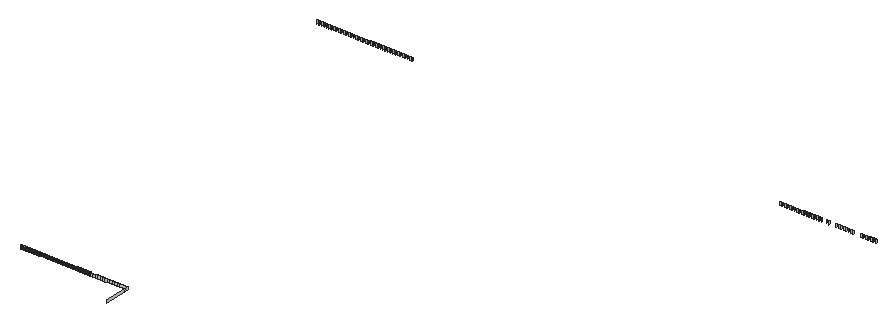
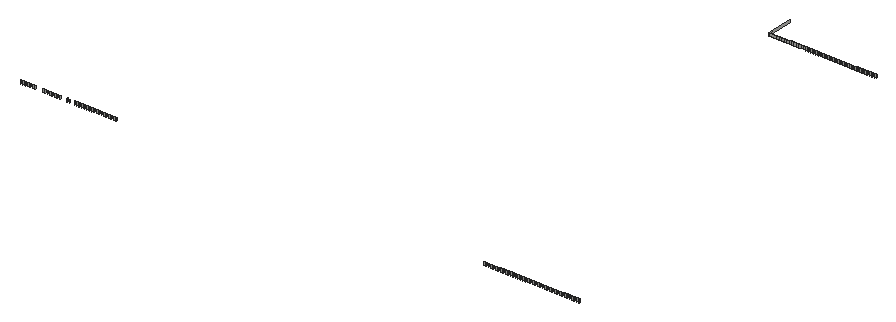
# SketchUp Ruby script. Lengths in inches.
U = 1.inch
M = Sketchup.active_model
def pt(a) = Geom::Point3d.new(a.map { |v| v * U })
def face(e, loops, mat)
  f = e.add_face(loops[0].map { |a| pt(a) })
  loops[1..].each { |l| e.add_face(l.map { |a| pt(a) }).erase! }
  f.material = f.back_material = mat if mat
  f
end
# faces: each face lists its corners as indices into pts; further lists are holes
def faces(e, pts, list, mat = nil) = list.each { |f| face(e, (f[0].is_a?(Array) ? f : [f]).map { |l| l.map { |i| pts[i] } }, mat) }
# xy, xz, yz: faces in a plane at the given z, y or x. An outline is a flat list of corners, or four numbers for a rectangle; further outlines are holes
def ring(l) = l.size == 4 ? [[l[0], l[1]], [l[2], l[1]], [l[2], l[3]], [l[0], l[3]]] : l.each_slice(2).to_a
def flat(e, list, mat, &to3) = list.each { |f| face(e, (f[0].is_a?(Array) ? f : [f]).map { |l| ring(l).map { |u, v| to3.(u, v) } }, mat) }
def xy(e, z, list, mat = nil) = flat(e, list, mat) { |x, y| [x, y, z] }
def xz(e, y, list, mat = nil) = flat(e, list, mat) { |x, z| [x, y, z] }
def yz(e, x, list, mat = nil) = flat(e, list, mat) { |y, z| [x, y, z] }
def lines(e, pts, list) = list.each { |a, b| e.add_line(pt(pts[a]), pt(pts[b])) }
# prism: a flat outline (further loops are holes) pulled along v
def prism(e, loops, v, mat = nil)
  f = face(e, loops, mat); d = Geom::Vector3d.new(v.map { |x| x * U })
  f.pushpull(f.normal.samedirection?(d) ? d.length : -d.length)
end
def box(e, o, s, mat = nil) = prism(e, [[o, [o[0] + s[0], o[1], o[2]], [o[0] + s[0], o[1] + s[1], o[2]], [o[0], o[1] + s[1], o[2]]]], [0, 0, s[2]], mat)
def at(x, y, z, deg = 0) = Geom::Transformation.translation(pt([x, y, z])) * Geom::Transformation.rotation(ORIGIN, Z_AXIS, deg.degrees)
def axes(o, x, y, z) = Geom::Transformation.new([*x, 0, *y, 0, *z, 0, *pt(o).to_a, 1])
def part(name) = M.definitions.add(name)
# library, detail: a bought-in or finely detailed component or shape, given as its bounding box
def library(name, o, s) = part(name).tap { |d| box(d.entities, o, s) }
def detail(e, o, s) = box(e.add_group.entities, o, s)
def put(e, d, t, mat = nil) = e.add_instance(d, t).tap { |i| i.material = mat if mat }
def group(e, t, mat = nil) = e.add_group.tap { |g| g.transformation = t; g.material = mat if mat }.entities
root = M.entities
xz(root,203.875,[[1539,-12.3125,1540.625,-8],[1541.375,-12.3125,1544.625,-8],[1545.375,-12.3125,1548.625,-8],[1549.375,-12.3125,1552.625,-8],[1553.375,-12.3125,1556.625,-8],
  [1557.375,-12.3125,1560.625,-8],[1561.375,-12.3125,1564.625,-8],[1565.375,-12.3125,1568.625,-8],[1569.375,-12.3125,1572.625,-8],[1573.375,-12.3125,1576.625,-8],
  [1577.375,-12.3125,1580.625,-8],[1581.375,-12.3125,1584.625,-8],[1585.375,-12.3125,1588.625,-8],[1589.375,-12.3125,1592.625,-8],[1593.375,-12.3125,1596.625,-8],
  [1597.375,-12.3125,1600.625,-8],[1601.375,-12.3125,1604.625,-8],[1605.375,-12.3125,1608.625,-8],[1609.375,-12.3125,1612.625,-8],[1613.375,-12.3125,1616.625,-8],
  [1617.375,-12.3125,1620.625,-8],[1621.375,-12.3125,1624.625,-8],[1625.375,-12.3125,1628.625,-8],[1629.375,-12.3125,1632.625,-8],[1633.375,-12.3125,1636.625,-8],
  [1637.375,-12.3125,1640.625,-8],[1641.375,-12.3125,1644.625,-8],[1645.375,-12.3125,1648.625,-8],[1649.375,-12.3125,1652.625,-8],[1653.375,-12.3125,1656.625,-8],
  [1657.375,-12.3125,1660.625,-8],[1661.375,-12.3125,1664.625,-8],[1665.375,-12.3125,1668.625,-8],[1669.375,-12.3125,1672.625,-8],[1673.375,-12.3125,1676.625,-8],
  [1677.375,-12.3125,1680.625,-8],[1681.375,-12.3125,1684.625,-8],[1685.375,-12.3125,1688.625,-8],[1689.375,-12.3125,1692.625,-8],[1693.375,-12.3125,1696.625,-8],
  [1697.375,-12.3125,1700.625,-8],[1700.625,-12.3125,1713.52,-8]])
xz(root,204.875,[[1540.625,-12.3125,1541.375,-8],[1544.625,-12.3125,1545.375,-8],[1548.625,-12.3125,1549.375,-8],[1552.625,-12.3125,1553.375,-8],[1556.625,-12.3125,1557.375,-8],
  [1560.625,-12.3125,1561.375,-8],[1564.625,-12.3125,1565.375,-8],[1568.625,-12.3125,1569.375,-8],[1572.625,-12.3125,1573.375,-8],[1576.625,-12.3125,1577.375,-8],
  [1580.625,-12.3125,1581.375,-8],[1584.625,-12.3125,1585.375,-8],[1588.625,-12.3125,1589.375,-8],[1592.625,-12.3125,1593.375,-8],[1596.625,-12.3125,1597.375,-8],
  [1600.625,-12.3125,1601.375,-8],[1604.625,-12.3125,1605.375,-8],[1608.625,-12.3125,1609.375,-8],[1612.625,-12.3125,1613.375,-8],[1616.625,-12.3125,1617.375,-8],
  [1620.625,-12.3125,1621.375,-8],[1624.625,-12.3125,1625.375,-8],[1628.625,-12.3125,1629.375,-8],[1632.625,-12.3125,1633.375,-8],[1636.625,-12.3125,1637.375,-8],
  [1640.625,-12.3125,1641.375,-8],[1644.625,-12.3125,1645.375,-8],[1648.625,-12.3125,1649.375,-8],[1652.625,-12.3125,1653.375,-8]])
xz(root,895.77,[[1468.9375,-12.3125,1469.6875,-8],[1472.9375,-12.3125,1473.6875,-8],[1476.9375,-12.3125,1477.6875,-8],[1480.9375,-12.3125,1481.6875,-8],[1484.9375,-12.3125,1485.6875,-8],
  [1488.9375,-12.3125,1489.6875,-8],[1492.9375,-12.3125,1493.6875,-8],[1496.9375,-12.3125,1497.6875,-8],[1500.9375,-12.3125,1501.6875,-8],[1504.9375,-12.3125,1505.6875,-8],
  [1508.9375,-12.3125,1509.6875,-8],[1512.9375,-12.3125,1513.6875,-8],[1516.9375,-12.3125,1517.6875,-8],[1520.9375,-12.3125,1521.6875,-8],[1524.9375,-12.3125,1525.6875,-8],
  [1528.9375,-12.3125,1529.6875,-8],[1532.9375,-12.3125,1533.6875,-8],[1536.9375,-12.3125,1537.6875,-8],[1540.9375,-12.3125,1541.6875,-8],[1544.9375,-12.3125,1545.6875,-8],
  [1548.9375,-12.3125,1549.6875,-8],[1552.9375,-12.3125,1553.6875,-8],[1556.9375,-12.3125,1557.6875,-8],[1560.9375,-12.3125,1561.6875,-8],[1564.9375,-12.3125,1565.6875,-8],
  [1568.9375,-12.3125,1569.6875,-8],[1572.9375,-12.3125,1573.6875,-8],[1576.9375,-12.3125,1577.6875,-8],[1580.9375,-12.3125,1581.6875,-8],[1584.9375,-12.3125,1585.6875,-8],
  [1588.9375,-12.3125,1589.6875,-8],[1592.9375,-12.3125,1593.6875,-8],[1596.9375,-12.3125,1597.6875,-8],[1600.9375,-12.3125,1601.6875,-8],[1604.9375,-12.3125,1605.6875,-8],
  [1608.9375,-12.3125,1609.6875,-8],[1612.9375,-12.3125,1613.6875,-8],[1616.9375,-12.3125,1617.6875,-8],[1620.9375,-12.3125,1621.6875,-8],[1624.9375,-12.3125,1625.6875,-8],
  [2223.5625,-12.3125,2224.3125,-8],[2227.5625,-12.3125,2228.3125,-8],[2231.5625,-12.3125,2232.3125,-8],[2235.5625,-12.3125,2236.3125,-8],[2239.5625,-12.3125,2240.3125,-8],
  [2243.5625,-12.3125,2244.3125,-8],[2247.5625,-12.3125,2248.3125,-8],[2251.5625,-12.3125,2252.3125,-8],[2255.5625,-12.3125,2256.3125,-8],[2259.5625,-12.3125,2260.3125,-8],
  [2263.5625,-12.3125,2264.3125,-8],[2267.5625,-12.3125,2268.3125,-8],[2271.5625,-12.3125,2272.3125,-8],[2275.5625,-12.3125,2276.3125,-8],[2279.5625,-12.3125,2280.3125,-8],
  [2283.5625,-12.3125,2284.3125,-8],[2287.5625,-12.3125,2288.3125,-8],[2299.5625,-12.3125,2300.3125,-8],[2303.5625,-12.3125,2304.3125,-8],[2319.5625,-12.3125,2320.3125,-8],
  [2327.5625,-12.3125,2328.3125,-8],[2359.5625,-12.3125,2360.3125,-8],[2363.5625,-12.3125,2364.3125,-8],[2367.5625,-12.3125,2368.3125,-8],[2371.5625,-12.3125,2372.3125,-8],
  [2375.5625,-12.3125,2376.3125,-8],[2379.5625,-12.3125,2380.3125,-8]])
yz(root,1468.9375,[[894.77,-12.3125,895.77,-8]])
yz(root,1469.6875,[[894.77,-12.3125,895.77,-8]])
yz(root,1472.9375,[[894.77,-12.3125,895.77,-8]])
yz(root,1473.6875,[[894.77,-12.3125,895.77,-8]])
yz(root,1476.9375,[[894.77,-12.3125,895.77,-8]])
yz(root,1477.6875,[[894.77,-12.3125,895.77,-8]])
yz(root,1480.9375,[[894.77,-12.3125,895.77,-8]])
yz(root,1481.6875,[[894.77,-12.3125,895.77,-8]])
yz(root,1484.9375,[[894.77,-12.3125,895.77,-8]])
yz(root,1485.6875,[[894.77,-12.3125,895.77,-8]])
yz(root,1488.9375,[[894.77,-12.3125,895.77,-8]])
yz(root,1489.6875,[[894.77,-12.3125,895.77,-8]])
yz(root,1492.9375,[[894.77,-12.3125,895.77,-8]])
yz(root,1493.6875,[[894.77,-12.3125,895.77,-8]])
yz(root,1496.9375,[[894.77,-12.3125,895.77,-8]])
yz(root,1497.6875,[[894.77,-12.3125,895.77,-8]])
yz(root,1500.9375,[[894.77,-12.3125,895.77,-8]])
yz(root,1501.6875,[[894.77,-12.3125,895.77,-8]])
yz(root,1504.9375,[[894.77,-12.3125,895.77,-8]])
yz(root,1505.6875,[[894.77,-12.3125,895.77,-8]])
yz(root,1508.9375,[[894.77,-12.3125,895.77,-8]])
yz(root,1509.6875,[[894.77,-12.3125,895.77,-8]])
yz(root,1512.9375,[[894.77,-12.3125,895.77,-8]])
yz(root,1513.6875,[[894.77,-12.3125,895.77,-8]])
yz(root,1516.9375,[[894.77,-12.3125,895.77,-8]])
yz(root,1517.6875,[[894.77,-12.3125,895.77,-8]])
yz(root,1520.9375,[[894.77,-12.3125,895.77,-8]])
yz(root,1521.6875,[[894.77,-12.3125,895.77,-8]])
yz(root,1524.9375,[[894.77,-12.3125,895.77,-8]])
yz(root,1525.6875,[[894.77,-12.3125,895.77,-8]])
yz(root,1528.9375,[[894.77,-12.3125,895.77,-8]])
yz(root,1529.6875,[[894.77,-12.3125,895.77,-8]])
yz(root,1532.9375,[[894.77,-12.3125,895.77,-8]])
yz(root,1533.6875,[[894.77,-12.3125,895.77,-8]])
yz(root,1536.9375,[[894.77,-12.3125,895.77,-8]])
yz(root,1537.6875,[[894.77,-12.3125,895.77,-8]])
yz(root,1540.625,[[203.875,-12.3125,204.875,-8]])
yz(root,1540.9375,[[894.77,-12.3125,895.77,-8]])
yz(root,1541.375,[[203.875,-12.3125,204.875,-8]])
yz(root,1541.6875,[[894.77,-12.3125,895.77,-8]])
yz(root,1544.625,[[203.875,-12.3125,204.875,-8]])
yz(root,1544.9375,[[894.77,-12.3125,895.77,-8]])
yz(root,1545.375,[[203.875,-12.3125,204.875,-8]])
yz(root,1545.6875,[[894.77,-12.3125,895.77,-8]])
yz(root,1548.625,[[203.875,-12.3125,204.875,-8]])
yz(root,1548.9375,[[894.77,-12.3125,895.77,-8]])
yz(root,1549.375,[[203.875,-12.3125,204.875,-8]])
yz(root,1549.6875,[[894.77,-12.3125,895.77,-8]])
yz(root,1552.625,[[203.875,-12.3125,204.875,-8]])
yz(root,1552.9375,[[894.77,-12.3125,895.77,-8]])
yz(root,1553.375,[[203.875,-12.3125,204.875,-8]])
yz(root,1553.6875,[[894.77,-12.3125,895.77,-8]])
yz(root,1556.625,[[203.875,-12.3125,204.875,-8]])
yz(root,1556.9375,[[894.77,-12.3125,895.77,-8]])
yz(root,1557.375,[[203.875,-12.3125,204.875,-8]])
yz(root,1557.6875,[[894.77,-12.3125,895.77,-8]])
yz(root,1560.625,[[203.875,-12.3125,204.875,-8]])
yz(root,1560.9375,[[894.77,-12.3125,895.77,-8]])
yz(root,1561.375,[[203.875,-12.3125,204.875,-8]])
yz(root,1561.6875,[[894.77,-12.3125,895.77,-8]])
yz(root,1564.625,[[203.875,-12.3125,204.875,-8]])
yz(root,1564.9375,[[894.77,-12.3125,895.77,-8]])
yz(root,1565.375,[[203.875,-12.3125,204.875,-8]])
yz(root,1565.6875,[[894.77,-12.3125,895.77,-8]])
yz(root,1568.625,[[203.875,-12.3125,204.875,-8]])
yz(root,1568.9375,[[894.77,-12.3125,895.77,-8]])
yz(root,1569.375,[[203.875,-12.3125,204.875,-8]])
yz(root,1569.6875,[[894.77,-12.3125,895.77,-8]])
yz(root,1572.625,[[203.875,-12.3125,204.875,-8]])
yz(root,1572.9375,[[894.77,-12.3125,895.77,-8]])
yz(root,1573.375,[[203.875,-12.3125,204.875,-8]])
yz(root,1573.6875,[[894.77,-12.3125,895.77,-8]])
yz(root,1576.625,[[203.875,-12.3125,204.875,-8]])
yz(root,1576.9375,[[894.77,-12.3125,895.77,-8]])
yz(root,1577.375,[[203.875,-12.3125,204.875,-8]])
yz(root,1577.6875,[[894.77,-12.3125,895.77,-8]])
yz(root,1580.625,[[203.875,-12.3125,204.875,-8]])
yz(root,1580.9375,[[894.77,-12.3125,895.77,-8]])
yz(root,1581.375,[[203.875,-12.3125,204.875,-8]])
yz(root,1581.6875,[[894.77,-12.3125,895.77,-8]])
yz(root,1584.625,[[203.875,-12.3125,204.875,-8]])
yz(root,1584.9375,[[894.77,-12.3125,895.77,-8]])
yz(root,1585.375,[[203.875,-12.3125,204.875,-8]])
yz(root,1585.6875,[[894.77,-12.3125,895.77,-8]])
yz(root,1588.625,[[203.875,-12.3125,204.875,-8]])
yz(root,1588.9375,[[894.77,-12.3125,895.77,-8]])
yz(root,1589.375,[[203.875,-12.3125,204.875,-8]])
yz(root,1589.6875,[[894.77,-12.3125,895.77,-8]])
yz(root,1592.625,[[203.875,-12.3125,204.875,-8]])
yz(root,1592.9375,[[894.77,-12.3125,895.77,-8]])
yz(root,1593.375,[[203.875,-12.3125,204.875,-8]])
yz(root,1593.6875,[[894.77,-12.3125,895.77,-8]])
yz(root,1596.625,[[203.875,-12.3125,204.875,-8]])
yz(root,1596.9375,[[894.77,-12.3125,895.77,-8]])
yz(root,1597.375,[[203.875,-12.3125,204.875,-8]])
yz(root,1597.6875,[[894.77,-12.3125,895.77,-8]])
yz(root,1600.625,[[203.875,-12.3125,204.875,-8]])
yz(root,1600.9375,[[894.77,-12.3125,895.77,-8]])
yz(root,1601.375,[[203.875,-12.3125,204.875,-8]])
yz(root,1601.6875,[[894.77,-12.3125,895.77,-8]])
yz(root,1604.625,[[203.875,-12.3125,204.875,-8]])
yz(root,1604.9375,[[894.77,-12.3125,895.77,-8]])
yz(root,1605.375,[[203.875,-12.3125,204.875,-8]])
yz(root,1605.6875,[[894.77,-12.3125,895.77,-8]])
yz(root,1608.625,[[203.875,-12.3125,204.875,-8]])
yz(root,1608.9375,[[894.77,-12.3125,895.77,-8]])
yz(root,1609.375,[[203.875,-12.3125,204.875,-8]])
yz(root,1609.6875,[[894.77,-12.3125,895.77,-8]])
yz(root,1612.625,[[203.875,-12.3125,204.875,-8]])
yz(root,1612.9375,[[894.77,-12.3125,895.77,-8]])
yz(root,1613.375,[[203.875,-12.3125,204.875,-8]])
yz(root,1613.6875,[[894.77,-12.3125,895.77,-8]])
yz(root,1616.625,[[203.875,-12.3125,204.875,-8]])
yz(root,1616.9375,[[894.77,-12.3125,895.77,-8]])
yz(root,1617.375,[[203.875,-12.3125,204.875,-8]])
yz(root,1617.6875,[[894.77,-12.3125,895.77,-8]])
yz(root,1620.625,[[203.875,-12.3125,204.875,-8]])
yz(root,1620.9375,[[894.77,-12.3125,895.77,-8]])
yz(root,1621.375,[[203.875,-12.3125,204.875,-8]])
yz(root,1621.6875,[[894.77,-12.3125,895.77,-8]])
yz(root,1624.625,[[203.875,-12.3125,204.875,-8]])
yz(root,1624.9375,[[894.77,-12.3125,895.77,-8]])
yz(root,1625.375,[[203.875,-12.3125,204.875,-8]])
yz(root,1625.6875,[[894.77,-12.3125,895.77,-8]])
yz(root,1628.625,[[203.875,-12.3125,204.875,-8]])
yz(root,1629.375,[[203.875,-12.3125,204.875,-8]])
yz(root,1632.625,[[203.875,-12.3125,204.875,-8]])
yz(root,1633.375,[[203.875,-12.3125,204.875,-8]])
yz(root,1636.625,[[203.875,-12.3125,204.875,-8]])
yz(root,1637.375,[[203.875,-12.3125,204.875,-8]])
yz(root,1640.625,[[203.875,-12.3125,204.875,-8]])
yz(root,1641.375,[[203.875,-12.3125,204.875,-8]])
yz(root,1644.625,[[203.875,-12.3125,204.875,-8]])
yz(root,1645.375,[[203.875,-12.3125,204.875,-8]])
yz(root,1648.625,[[203.875,-12.3125,204.875,-8]])
yz(root,1649.375,[[203.875,-12.3125,204.875,-8]])
yz(root,1652.625,[[203.875,-12.3125,204.875,-8]])
yz(root,1713.52,[[162.33,-12.3125,198.625,-8],[198.625,-12.3125,203.875,-8]])
yz(root,2223.5625,[[894.77,-12.3125,895.77,-8]])
yz(root,2224.3125,[[894.77,-12.3125,895.77,-8]])
yz(root,2227.5625,[[894.77,-12.3125,895.77,-8]])
yz(root,2228.3125,[[894.77,-12.3125,895.77,-8]])
yz(root,2231.5625,[[894.77,-12.3125,895.77,-8]])
yz(root,2232.3125,[[894.77,-12.3125,895.77,-8]])
yz(root,2235.5625,[[894.77,-12.3125,895.77,-8]])
yz(root,2236.3125,[[894.77,-12.3125,895.77,-8]])
yz(root,2239.5625,[[894.77,-12.3125,895.77,-8]])
yz(root,2240.3125,[[894.77,-12.3125,895.77,-8]])
yz(root,2243.5625,[[894.77,-12.3125,895.77,-8]])
yz(root,2244.3125,[[894.77,-12.3125,895.77,-8]])
yz(root,2247.5625,[[894.77,-12.3125,895.77,-8]])
yz(root,2248.3125,[[894.77,-12.3125,895.77,-8]])
yz(root,2251.5625,[[894.77,-12.3125,895.77,-8]])
yz(root,2252.3125,[[894.77,-12.3125,895.77,-8]])
yz(root,2255.5625,[[894.77,-12.3125,895.77,-8]])
yz(root,2256.3125,[[894.77,-12.3125,895.77,-8]])
yz(root,2259.5625,[[894.77,-12.3125,895.77,-8]])
yz(root,2260.3125,[[894.77,-12.3125,895.77,-8]])
yz(root,2263.5625,[[894.77,-12.3125,895.77,-8]])
yz(root,2264.3125,[[894.77,-12.3125,895.77,-8]])
yz(root,2267.5625,[[894.77,-12.3125,895.77,-8]])
yz(root,2271.5625,[[894.77,-12.3125,895.77,-8]])
yz(root,2272.3125,[[894.77,-12.3125,895.77,-8]])
yz(root,2275.5625,[[894.77,-12.3125,895.77,-8]])
yz(root,2276.3125,[[894.77,-12.3125,895.77,-8]])
yz(root,2279.5625,[[894.77,-12.3125,895.77,-8]])
yz(root,2280.3125,[[894.77,-12.3125,895.77,-8]])
yz(root,2283.5625,[[894.77,-12.3125,895.77,-8]])
yz(root,2284.3125,[[894.77,-12.3125,895.77,-8]])
yz(root,2287.5625,[[894.77,-12.3125,895.77,-8]])
yz(root,2288.3125,[[894.77,-12.3125,895.77,-8]])
yz(root,2292.3125,[[894.77,-12.3125,895.77,-8]])
yz(root,2303.5625,[[894.77,-12.3125,895.77,-8]])
yz(root,2304.3125,[[894.77,-12.3125,895.77,-8]])
yz(root,2315.5625,[[894.77,-12.3125,895.77,-8]])
yz(root,2320.3125,[[894.77,-12.3125,895.77,-8]])
yz(root,2323.5625,[[894.77,-12.3125,895.77,-8]])
yz(root,2327.5625,[[894.77,-12.3125,895.77,-8]])
yz(root,2328.3125,[[894.77,-12.3125,895.77,-8]])
yz(root,2331.5625,[[894.77,-12.3125,895.77,-8]])
yz(root,2335.5625,[[894.77,-12.3125,895.77,-8]])
yz(root,2340.3125,[[894.77,-12.3125,895.77,-8]])
yz(root,2343.5625,[[894.77,-12.3125,895.77,-8]])
yz(root,2356.3125,[[894.77,-12.3125,895.77,-8]])
yz(root,2359.5625,[[894.77,-12.3125,895.77,-8]])
yz(root,2360.3125,[[894.77,-12.3125,895.77,-8]])
yz(root,2363.5625,[[894.77,-12.3125,895.77,-8]])
yz(root,2364.3125,[[894.77,-12.3125,895.77,-8]])
yz(root,2367.5625,[[894.77,-12.3125,895.77,-8]])
yz(root,2368.3125,[[894.77,-12.3125,895.77,-8]])
yz(root,2371.5625,[[894.77,-12.3125,895.77,-8]])
yz(root,2372.3125,[[894.77,-12.3125,895.77,-8]])
yz(root,2375.5625,[[894.77,-12.3125,895.77,-8]])
yz(root,2376.3125,[[894.77,-12.3125,895.77,-8]])
yz(root,2379.5625,[[894.77,-12.3125,895.77,-8]])
yz(root,2380.3125,[[894.77,-12.3125,895.77,-8]])
